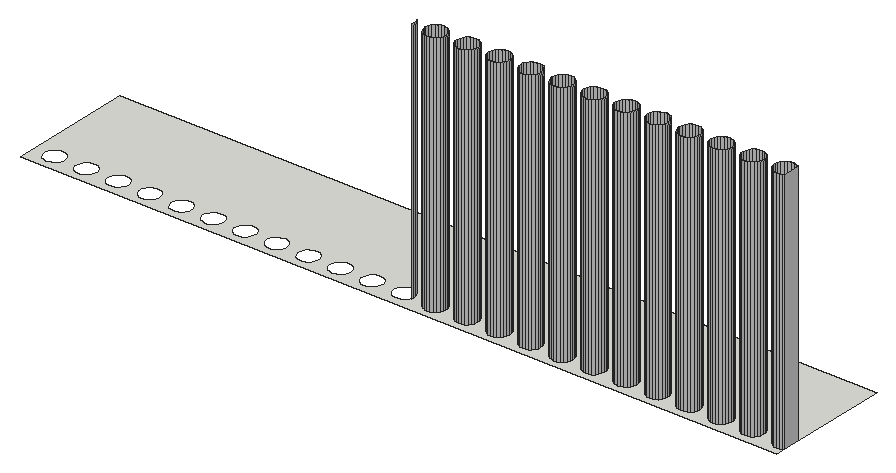
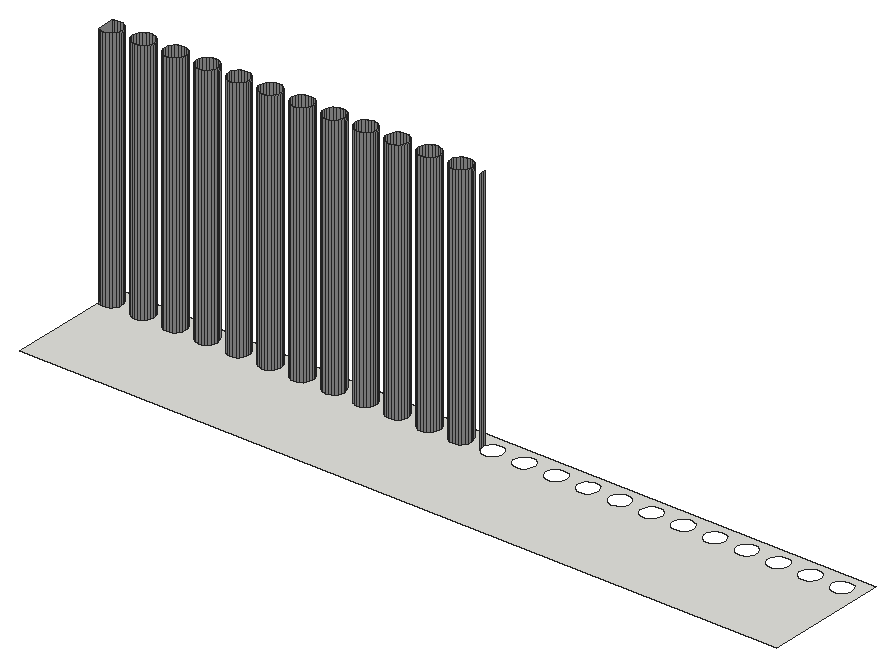
# SketchUp Ruby script. Lengths in millimetres.
U = 1.mm
M = Sketchup.active_model
def pt(a) = Geom::Point3d.new(a.map { |v| v * U })
def face(e, loops, mat)
  f = e.add_face(loops[0].map { |a| pt(a) })
  loops[1..].each { |l| e.add_face(l.map { |a| pt(a) }).erase! }
  f.material = f.back_material = mat if mat
  f
end
# faces: each face lists its corners as indices into pts; further lists are holes
def faces(e, pts, list, mat = nil) = list.each { |f| face(e, (f[0].is_a?(Array) ? f : [f]).map { |l| l.map { |i| pts[i] } }, mat) }
# xy, xz, yz: faces in a plane at the given z, y or x. An outline is a flat list of corners, or four numbers for a rectangle; further outlines are holes
def ring(l) = l.size == 4 ? [[l[0], l[1]], [l[2], l[1]], [l[2], l[3]], [l[0], l[3]]] : l.each_slice(2).to_a
def flat(e, list, mat, &to3) = list.each { |f| face(e, (f[0].is_a?(Array) ? f : [f]).map { |l| ring(l).map { |u, v| to3.(u, v) } }, mat) }
def xy(e, z, list, mat = nil) = flat(e, list, mat) { |x, y| [x, y, z] }
def xz(e, y, list, mat = nil) = flat(e, list, mat) { |x, z| [x, y, z] }
def yz(e, x, list, mat = nil) = flat(e, list, mat) { |y, z| [x, y, z] }
def lines(e, pts, list) = list.each { |a, b| e.add_line(pt(pts[a]), pt(pts[b])) }
# prism: a flat outline (further loops are holes) pulled along v
def prism(e, loops, v, mat = nil)
  f = face(e, loops, mat); d = Geom::Vector3d.new(v.map { |x| x * U })
  f.pushpull(f.normal.samedirection?(d) ? d.length : -d.length)
end
def box(e, o, s, mat = nil) = prism(e, [[o, [o[0] + s[0], o[1], o[2]], [o[0] + s[0], o[1] + s[1], o[2]], [o[0], o[1] + s[1], o[2]]]], [0, 0, s[2]], mat)
def at(x, y, z, deg = 0) = Geom::Transformation.translation(pt([x, y, z])) * Geom::Transformation.rotation(ORIGIN, Z_AXIS, deg.degrees)
def axes(o, x, y, z) = Geom::Transformation.new([*x, 0, *y, 0, *z, 0, *pt(o).to_a, 1])
def part(name) = M.definitions.add(name)
# library, detail: a bought-in or finely detailed component or shape, given as its bounding box
def library(name, o, s) = part(name).tap { |d| box(d.entities, o, s) }
def detail(e, o, s) = box(e.add_group.entities, o, s)
def put(e, d, t, mat = nil) = e.add_instance(d, t).tap { |i| i.material = mat if mat }
def group(e, t, mat = nil) = e.add_group.tap { |g| g.transformation = t; g.material = mat if mat }.entities
root = M.entities
M.materials.add("[Metal Corrugated Shiny]").color = [193, 193, 193]
xy(root,3899.4,[[[7199.4,887.4,11890.5,887.4,11890.5,946.6,11883.2,941.2,11867.4,934.9,11850.5,932.9,11833.7,935.4,11818.1,942.1,11804.8,952.6,11794.6,966.2,11788.3,982,11786.4,998.9,11788.8,1015.7,11795.5,1031.3,11806.1,1044.7,11819.7,1054.8,11835.5,1061.1,11852.3,1063.1,11869.2,1060.6,11884.8,1053.9,11890.5,1049.4,11890.5,1657.4,7199.4,1657.4],[11063.1,932.9,11046.3,935.4,11030.7,942.1,11017.4,952.6,11007.2,966.2,11000.9,982,10999,998.9,11001.4,1015.7,11008.1,1031.3,11018.7,1044.7,11032.3,1054.8,11048.1,1061.1,11064.9,1063.1,11081.8,1060.6,11097.4,1053.9,11110.7,1043.4,11120.9,1029.8,11127.1,1014,11129.1,997.1,11126.7,980.3,11120,964.7,11109.4,951.3,11095.8,941.2,11080,934.9],[11653.7,932.9,11636.9,935.4,11621.3,942.1,11607.9,952.6,11597.8,966.2,11591.5,982,11589.5,998.9,11592,1015.7,11598.7,1031.3,11609.2,1044.7,11622.8,1054.8,11638.6,1061.1,11655.5,1063.1,11672.3,1060.6,11687.9,1053.9,11701.3,1043.4,11711.4,1029.8,11717.7,1014,11719.7,997.1,11717.2,980.3,11710.5,964.7,11700,951.3,11686.4,941.2,11670.6,934.9],[11260,932.9,11243.2,935.4,11227.6,942.1,11214.2,952.6,11204.1,966.2,11197.8,982,11195.8,998.9,11198.3,1015.7,11205,1031.3,11215.5,1044.7,11229.1,1054.8,11244.9,1061.1,11261.8,1063.1,11278.6,1060.6,11294.2,1053.9,11307.6,1043.4,11317.7,1029.8,11324,1014,11326,997.1,11323.5,980.3,11316.8,964.7,11306.3,951.3,11292.7,941.2,11276.9,934.9],[10669.4,932.9,10652.6,935.4,10637,942.1,10623.7,952.6,10613.5,966.2,10607.2,982,10605.3,998.9,10607.7,1015.7,10614.4,1031.3,10625,1044.7,10638.6,1054.8,10654.4,1061.1,10671.2,1063.1,10688.1,1060.6,10703.7,1053.9,10717,1043.4,10727.2,1029.8,10733.4,1014,10735.4,997.1,10733,980.3,10726.3,964.7,10715.7,951.3,10702.1,941.2,10686.3,934.9],[8110.4,932.9,8093.6,935.4,8078,942.1,8064.6,952.6,8054.5,966.2,8048.2,982,8046.2,998.9,8048.7,1015.7,8055.4,1031.3,8065.9,1044.7,8079.5,1054.8,8095.3,1061.1,8112.2,1063.1,8129,1060.6,8144.6,1053.9,8158,1043.4,8168.1,1029.8,8174.4,1014,8176.4,997.1,8173.9,980.3,8167.2,964.7,8156.7,951.3,8143.1,941.2,8127.3,934.9],[9882,932.9,9865.2,935.4,9849.6,942.1,9836.3,952.6,9826.1,966.2,9819.8,982,9817.9,998.9,9820.3,1015.7,9827,1031.3,9837.6,1044.7,9851.2,1054.8,9867,1061.1,9883.8,1063.1,9900.7,1060.6,9916.3,1053.9,9929.6,1043.4,9939.8,1029.8,9946,1014,9948,997.1,9945.6,980.3,9938.9,964.7,9928.3,951.3,9914.7,941.2,9898.9,934.9],[11456.8,932.9,11440,935.4,11424.4,942.1,11411.1,952.6,11400.9,966.2,11394.6,982,11392.7,998.9,11395.1,1015.7,11401.8,1031.3,11412.4,1044.7,11426,1054.8,11441.8,1061.1,11458.6,1063.1,11475.5,1060.6,11491.1,1053.9,11504.4,1043.4,11514.6,1029.8,11520.8,1014,11522.8,997.1,11520.4,980.3,11513.7,964.7,11503.1,951.3,11489.5,941.2,11473.7,934.9],[7323,932.9,7306.2,935.4,7290.6,942.1,7277.2,952.6,7267.1,966.2,7260.8,982,7258.8,998.9,7261.3,1015.7,7268,1031.3,7278.5,1044.7,7292.1,1054.8,7307.9,1061.1,7324.8,1063.1,7341.6,1060.6,7357.2,1053.9,7370.6,1043.4,7380.7,1029.8,7387,1014,7389,997.1,7386.5,980.3,7379.8,964.7,7369.3,951.3,7355.7,941.2,7339.9,934.9],[7716.7,932.9,7699.9,935.4,7684.3,942.1,7670.9,952.6,7660.8,966.2,7654.5,982,7652.5,998.9,7655,1015.7,7661.7,1031.3,7672.2,1044.7,7685.8,1054.8,7701.6,1061.1,7718.5,1063.1,7735.3,1060.6,7750.9,1053.9,7764.3,1043.4,7774.4,1029.8,7780.7,1014,7782.7,997.1,7780.2,980.3,7773.5,964.7,7763,951.3,7749.4,941.2,7733.6,934.9],[7913.5,932.9,7896.7,935.4,7881.1,942.1,7867.8,952.6,7857.6,966.2,7851.3,982,7849.4,998.9,7851.8,1015.7,7858.5,1031.3,7869.1,1044.7,7882.7,1054.8,7898.5,1061.1,7915.3,1063.1,7932.2,1060.6,7947.8,1053.9,7961.1,1043.4,7971.3,1029.8,7977.5,1014,7979.5,997.1,7977.1,980.3,7970.4,964.7,7959.8,951.3,7946.2,941.2,7930.4,934.9],[8897.8,932.9,8881,935.4,8865.4,942.1,8852,952.6,8841.9,966.2,8835.6,982,8833.6,998.9,8836.1,1015.7,8842.8,1031.3,8853.3,1044.7,8866.9,1054.8,8882.7,1061.1,8899.6,1063.1,8916.4,1060.6,8932,1053.9,8945.4,1043.4,8955.5,1029.8,8961.8,1014,8963.8,997.1,8961.3,980.3,8954.6,964.7,8944.1,951.3,8930.5,941.2,8914.7,934.9],[9094.6,932.9,9077.8,935.4,9062.2,942.1,9048.9,952.6,9038.7,966.2,9032.4,982,9030.5,998.9,9032.9,1015.7,9039.6,1031.3,9050.2,1044.7,9063.8,1054.8,9079.6,1061.1,9096.4,1063.1,9113.3,1060.6,9128.9,1053.9,9142.2,1043.4,9152.4,1029.8,9158.6,1014,9160.6,997.1,9158.2,980.3,9151.5,964.7,9140.9,951.3,9127.3,941.2,9111.5,934.9],[7519.8,932.9,7503,935.4,7487.4,942.1,7474.1,952.6,7463.9,966.2,7457.6,982,7455.7,998.9,7458.1,1015.7,7464.8,1031.3,7475.4,1044.7,7489,1054.8,7504.8,1061.1,7521.6,1063.1,7538.5,1060.6,7554.1,1053.9,7567.4,1043.4,7577.6,1029.8,7583.8,1014,7585.8,997.1,7583.4,980.3,7576.7,964.7,7566.1,951.3,7552.5,941.2,7536.7,934.9],[8504.1,932.9,8487.3,935.4,8471.7,942.1,8458.3,952.6,8448.2,966.2,8441.9,982,8439.9,998.9,8442.4,1015.7,8449.1,1031.3,8459.6,1044.7,8473.2,1054.8,8489,1061.1,8505.9,1063.1,8522.7,1060.6,8538.3,1053.9,8551.7,1043.4,8561.8,1029.8,8568.1,1014,8570.1,997.1,8567.6,980.3,8560.9,964.7,8550.4,951.3,8536.8,941.2,8521,934.9],[9488.3,932.9,9471.5,935.4,9455.9,942.1,9442.6,952.6,9432.4,966.2,9426.1,982,9424.2,998.9,9426.6,1015.7,9433.3,1031.3,9443.9,1044.7,9457.5,1054.8,9473.3,1061.1,9490.1,1063.1,9507,1060.6,9522.6,1053.9,9535.9,1043.4,9546.1,1029.8,9552.3,1014,9554.3,997.1,9551.9,980.3,9545.2,964.7,9534.6,951.3,9521,941.2,9505.2,934.9],[10472.6,932.9,10455.8,935.4,10440.2,942.1,10426.8,952.6,10416.7,966.2,10410.4,982,10408.4,998.9,10410.9,1015.7,10417.6,1031.3,10428.1,1044.7,10441.7,1054.8,10457.5,1061.1,10474.4,1063.1,10491.2,1060.6,10506.8,1053.9,10520.2,1043.4,10530.3,1029.8,10536.6,1014,10538.6,997.1,10536.1,980.3,10529.4,964.7,10518.9,951.3,10505.3,941.2,10489.5,934.9],[9685.2,932.9,9668.4,935.4,9652.8,942.1,9639.4,952.6,9629.3,966.2,9623,982,9621,998.9,9623.5,1015.7,9630.2,1031.3,9640.7,1044.7,9654.3,1054.8,9670.1,1061.1,9687,1063.1,9703.8,1060.6,9719.4,1053.9,9732.8,1043.4,9742.9,1029.8,9749.2,1014,9751.2,997.1,9748.7,980.3,9742,964.7,9731.5,951.3,9717.9,941.2,9702.1,934.9],[8700.9,932.9,8684.1,935.4,8668.5,942.1,8655.2,952.6,8645,966.2,8638.7,982,8636.8,998.9,8639.2,1015.7,8645.9,1031.3,8656.5,1044.7,8670.1,1054.8,8685.9,1061.1,8702.7,1063.1,8719.6,1060.6,8735.2,1053.9,8748.5,1043.4,8758.7,1029.8,8764.9,1014,8766.9,997.1,8764.5,980.3,8757.8,964.7,8747.2,951.3,8733.6,941.2,8717.8,934.9],[10078.9,932.9,10062.1,935.4,10046.5,942.1,10033.1,952.6,10023,966.2,10016.7,982,10014.7,998.9,10017.2,1015.7,10023.9,1031.3,10034.4,1044.7,10048,1054.8,10063.8,1061.1,10080.7,1063.1,10097.5,1060.6,10113.1,1053.9,10126.5,1043.4,10136.6,1029.8,10142.9,1014,10144.9,997.1,10142.4,980.3,10135.7,964.7,10125.2,951.3,10111.6,941.2,10095.8,934.9],[8307.2,932.9,8290.4,935.4,8274.8,942.1,8261.5,952.6,8251.3,966.2,8245,982,8243.1,998.9,8245.5,1015.7,8252.2,1031.3,8262.8,1044.7,8276.4,1054.8,8292.2,1061.1,8309,1063.1,8325.9,1060.6,8341.5,1053.9,8354.8,1043.4,8365,1029.8,8371.2,1014,8373.2,997.1,8370.8,980.3,8364.1,964.7,8353.5,951.3,8339.9,941.2,8324.1,934.9],[9291.5,932.9,9274.7,935.4,9259.1,942.1,9245.7,952.6,9235.6,966.2,9229.3,982,9227.3,998.9,9229.8,1015.7,9236.5,1031.3,9247,1044.7,9260.6,1054.8,9276.4,1061.1,9293.3,1063.1,9310.1,1060.6,9325.7,1053.9,9339.1,1043.4,9349.2,1029.8,9355.5,1014,9357.5,997.1,9355,980.3,9348.3,964.7,9337.8,951.3,9324.2,941.2,9308.4,934.9],[10275.7,932.9,10258.9,935.4,10243.3,942.1,10230,952.6,10219.8,966.2,10213.5,982,10211.6,998.9,10214,1015.7,10220.7,1031.3,10231.3,1044.7,10244.9,1054.8,10260.7,1061.1,10277.5,1063.1,10294.4,1060.6,10310,1053.9,10323.3,1043.4,10333.5,1029.8,10339.7,1014,10341.7,997.1,10339.3,980.3,10332.6,964.7,10322,951.3,10308.4,941.2,10292.6,934.9],[10866.3,932.9,10849.5,935.4,10833.9,942.1,10820.5,952.6,10810.4,966.2,10804.1,982,10802.1,998.9,10804.6,1015.7,10811.3,1031.3,10821.8,1044.7,10835.4,1054.8,10851.2,1061.1,10868.1,1063.1,10884.9,1060.6,10900.5,1053.9,10913.9,1043.4,10924,1029.8,10930.3,1014,10932.3,997.1,10929.8,980.3,10923.1,964.7,10912.6,951.3,10899,941.2,10883.2,934.9]]])
xy(root,3899.4,[[9685.2,932.9,9668.4,935.4,9652.8,942.1,9639.4,952.6,9629.3,966.2,9623,982,9621,998.9,9623.5,1015.7,9630.2,1031.3,9640.7,1044.7,9654.3,1054.8,9670.1,1061.1,9687,1063.1,9703.8,1060.6,9719.4,1053.9,9732.8,1043.4,9742.9,1029.8,9749.2,1014,9751.2,997.1,9748.7,980.3,9742,964.7,9731.5,951.3,9717.9,941.2,9702.1,934.9],[9882,932.9,9865.2,935.4,9849.6,942.1,9836.3,952.6,9826.1,966.2,9819.8,982,9817.9,998.9,9820.3,1015.7,9827,1031.3,9837.6,1044.7,9851.2,1054.8,9867,1061.1,9883.8,1063.1,9900.7,1060.6,9916.3,1053.9,9929.6,1043.4,9939.8,1029.8,9946,1014,9948,997.1,9945.6,980.3,9938.9,964.7,9928.3,951.3,9914.7,941.2,9898.9,934.9],[10078.9,932.9,10062.1,935.4,10046.5,942.1,10033.1,952.6,10023,966.2,10016.7,982,10014.7,998.9,10017.2,1015.7,10023.9,1031.3,10034.4,1044.7,10048,1054.8,10063.8,1061.1,10080.7,1063.1,10097.5,1060.6,10113.1,1053.9,10126.5,1043.4,10136.6,1029.8,10142.9,1014,10144.9,997.1,10142.4,980.3,10135.7,964.7,10125.2,951.3,10111.6,941.2,10095.8,934.9],[10275.7,932.9,10258.9,935.4,10243.3,942.1,10230,952.6,10219.8,966.2,10213.5,982,10211.6,998.9,10214,1015.7,10220.7,1031.3,10231.3,1044.7,10244.9,1054.8,10260.7,1061.1,10277.5,1063.1,10294.4,1060.6,10310,1053.9,10323.3,1043.4,10333.5,1029.8,10339.7,1014,10341.7,997.1,10339.3,980.3,10332.6,964.7,10322,951.3,10308.4,941.2,10292.6,934.9],[10472.6,932.9,10455.8,935.4,10440.2,942.1,10426.8,952.6,10416.7,966.2,10410.4,982,10408.4,998.9,10410.9,1015.7,10417.6,1031.3,10428.1,1044.7,10441.7,1054.8,10457.5,1061.1,10474.4,1063.1,10491.2,1060.6,10506.8,1053.9,10520.2,1043.4,10530.3,1029.8,10536.6,1014,10538.6,997.1,10536.1,980.3,10529.4,964.7,10518.9,951.3,10505.3,941.2,10489.5,934.9],
  [10669.4,932.9,10652.6,935.4,10637,942.1,10623.7,952.6,10613.5,966.2,10607.2,982,10605.3,998.9,10607.7,1015.7,10614.4,1031.3,10625,1044.7,10638.6,1054.8,10654.4,1061.1,10671.2,1063.1,10688.1,1060.6,10703.7,1053.9,10717,1043.4,10727.2,1029.8,10733.4,1014,10735.4,997.1,10733,980.3,10726.3,964.7,10715.7,951.3,10702.1,941.2,10686.3,934.9],[10866.3,932.9,10849.5,935.4,10833.9,942.1,10820.5,952.6,10810.4,966.2,10804.1,982,10802.1,998.9,10804.6,1015.7,10811.3,1031.3,10821.8,1044.7,10835.4,1054.8,10851.2,1061.1,10868.1,1063.1,10884.9,1060.6,10900.5,1053.9,10913.9,1043.4,10924,1029.8,10930.3,1014,10932.3,997.1,10929.8,980.3,10923.1,964.7,10912.6,951.3,10899,941.2,10883.2,934.9],[11063.1,932.9,11046.3,935.4,11030.7,942.1,11017.4,952.6,11007.2,966.2,11000.9,982,10999,998.9,11001.4,1015.7,11008.1,1031.3,11018.7,1044.7,11032.3,1054.8,11048.1,1061.1,11064.9,1063.1,11081.8,1060.6,11097.4,1053.9,11110.7,1043.4,11120.9,1029.8,11127.1,1014,11129.1,997.1,11126.7,980.3,11120,964.7,11109.4,951.3,11095.8,941.2,11080,934.9],[11260,932.9,11243.2,935.4,11227.6,942.1,11214.2,952.6,11204.1,966.2,11197.8,982,11195.8,998.9,11198.3,1015.7,11205,1031.3,11215.5,1044.7,11229.1,1054.8,11244.9,1061.1,11261.8,1063.1,11278.6,1060.6,11294.2,1053.9,11307.6,1043.4,11317.7,1029.8,11324,1014,11326,997.1,11323.5,980.3,11316.8,964.7,11306.3,951.3,11292.7,941.2,11276.9,934.9],[11456.8,932.9,11440,935.4,11424.4,942.1,11411.1,952.6,11400.9,966.2,11394.6,982,11392.7,998.9,11395.1,1015.7,11401.8,1031.3,11412.4,1044.7,11426,1054.8,11441.8,1061.1,11458.6,1063.1,11475.5,1060.6,11491.1,1053.9,11504.4,1043.4,11514.6,1029.8,11520.8,1014,11522.8,997.1,11520.4,980.3,11513.7,964.7,11503.1,951.3,11489.5,941.2,11473.7,934.9],
  [11653.7,932.9,11636.9,935.4,11621.3,942.1,11607.9,952.6,11597.8,966.2,11591.5,982,11589.5,998.9,11592,1015.7,11598.7,1031.3,11609.2,1044.7,11622.8,1054.8,11638.6,1061.1,11655.5,1063.1,11672.3,1060.6,11687.9,1053.9,11701.3,1043.4,11711.4,1029.8,11717.7,1014,11719.7,997.1,11717.2,980.3,11710.5,964.7,11700,951.3,11686.4,941.2,11670.6,934.9],[11850.5,932.9,11833.7,935.4,11818.1,942.1,11804.8,952.6,11794.6,966.2,11788.3,982,11786.4,998.9,11788.8,1015.7,11795.5,1031.3,11806.1,1044.7,11819.7,1054.8,11835.5,1061.1,11852.3,1063.1,11869.2,1060.6,11884.8,1053.9,11890.5,1049.4,11890.5,946.6,11883.2,941.2,11867.4,934.9]],"[Metal Corrugated Shiny]")
yz(root,11890.5,[[946.6,3899.4,1049.4,5423.4]],"[Metal Corrugated Shiny]")
p = [[9668.4,935.4,3899.4],[9685.2,932.9,3899.4],[9685.2,932.9,5423.4],[9668.4,935.4,5423.4],[9702.1,934.9,3899.4],[9702.1,934.9,5423.4],
  [9865.2,935.4,3899.4],[9882,932.9,3899.4],[9882,932.9,5423.4],[9865.2,935.4,5423.4],[9898.9,934.9,3899.4],[9898.9,934.9,5423.4],
  [10062.1,935.4,3899.4],[10078.9,932.9,3899.4],[10078.9,932.9,5423.4],[10062.1,935.4,5423.4],[10095.8,934.9,3899.4],[10095.8,934.9,5423.4],
  [10258.9,935.4,3899.4],[10275.7,932.9,3899.4],[10275.7,932.9,5423.4],[10258.9,935.4,5423.4],[10292.6,934.9,3899.4],[10292.6,934.9,5423.4],
  [10455.8,935.4,3899.4],[10472.6,932.9,3899.4],[10472.6,932.9,5423.4],[10455.8,935.4,5423.4],[10489.5,934.9,3899.4],[10489.5,934.9,5423.4],
  [10652.6,935.4,3899.4],[10669.4,932.9,3899.4],[10669.4,932.9,5423.4],[10652.6,935.4,5423.4],[10686.3,934.9,3899.4],[10686.3,934.9,5423.4],
  [10849.5,935.4,3899.4],[10866.3,932.9,3899.4],[10866.3,932.9,5423.4],[10849.5,935.4,5423.4],[10883.2,934.9,3899.4],[10883.2,934.9,5423.4],
  [11046.3,935.4,3899.4],[11063.1,932.9,3899.4],[11063.1,932.9,5423.4],[11046.3,935.4,5423.4],[11080,934.9,3899.4],[11080,934.9,5423.4],
  [11243.2,935.4,3899.4],[11260,932.9,3899.4],[11260,932.9,5423.4],[11243.2,935.4,5423.4],[11276.9,934.9,3899.4],[11276.9,934.9,5423.4],
  [11440,935.4,3899.4],[11456.8,932.9,3899.4],[11456.8,932.9,5423.4],[11440,935.4,5423.4],[11473.7,934.9,3899.4],[11473.7,934.9,5423.4],
  [11636.9,935.4,3899.4],[11653.7,932.9,3899.4],[11653.7,932.9,5423.4],[11636.9,935.4,5423.4],[11670.6,934.9,3899.4],[11670.6,934.9,5423.4],
  [11833.7,935.4,3899.4],[11850.5,932.9,3899.4],[11850.5,932.9,5423.4],[11833.7,935.4,5423.4],[11867.4,934.9,3899.4],[11867.4,934.9,5423.4],
  [9717.9,941.2,3899.4],[9717.9,941.2,5423.4],[9914.7,941.2,3899.4],[9914.7,941.2,5423.4],[10111.6,941.2,3899.4],[10111.6,941.2,5423.4],
  [10308.4,941.2,3899.4],[10308.4,941.2,5423.4],[10505.3,941.2,3899.4],[10505.3,941.2,5423.4],[10702.1,941.2,3899.4],[10702.1,941.2,5423.4],
  [10899,941.2,3899.4],[10899,941.2,5423.4],[11095.8,941.2,3899.4],[11095.8,941.2,5423.4],[11292.7,941.2,3899.4],[11292.7,941.2,5423.4],
  [11489.5,941.2,3899.4],[11489.5,941.2,5423.4],[11686.4,941.2,3899.4],[11686.4,941.2,5423.4],[11883.2,941.2,3899.4],[11883.2,941.2,5423.4],
  [9652.8,942.1,3899.4],[9652.8,942.1,5423.4],[9849.6,942.1,3899.4],[9849.6,942.1,5423.4],[10046.5,942.1,3899.4],[10046.5,942.1,5423.4],
  [10243.3,942.1,3899.4],[10243.3,942.1,5423.4],[10440.2,942.1,3899.4],[10440.2,942.1,5423.4],[10637,942.1,3899.4],[10637,942.1,5423.4],
  [10833.9,942.1,3899.4],[10833.9,942.1,5423.4],[11030.7,942.1,3899.4],[11030.7,942.1,5423.4],[11227.6,942.1,3899.4],[11227.6,942.1,5423.4],
  [11424.4,942.1,3899.4],[11424.4,942.1,5423.4],[11621.3,942.1,3899.4],[11621.3,942.1,5423.4],[11818.1,942.1,3899.4],[11818.1,942.1,5423.4],
  [9731.5,951.3,3899.4],[9731.5,951.3,5423.4],[9928.3,951.3,3899.4],[9928.3,951.3,5423.4],[10125.2,951.3,3899.4],[10125.2,951.3,5423.4],
  [10322,951.3,3899.4],[10322,951.3,5423.4],[10518.9,951.3,3899.4],[10518.9,951.3,5423.4],[10715.7,951.3,3899.4],[10715.7,951.3,5423.4],
  [10912.6,951.3,3899.4],[10912.6,951.3,5423.4],[11109.4,951.3,3899.4],[11109.4,951.3,5423.4],[11306.3,951.3,3899.4],[11306.3,951.3,5423.4],
  [11503.1,951.3,3899.4],[11503.1,951.3,5423.4],[11700,951.3,3899.4],[11700,951.3,5423.4],[11890.5,946.6,3899.4],[11890.5,946.6,5423.4],
  [9639.4,952.6,3899.4],[9639.4,952.6,5423.4],[9836.3,952.6,3899.4],[9836.3,952.6,5423.4],[10033.1,952.6,3899.4],[10033.1,952.6,5423.4],
  [10230,952.6,3899.4],[10230,952.6,5423.4],[10426.8,952.6,3899.4],[10426.8,952.6,5423.4],[10623.7,952.6,3899.4],[10623.7,952.6,5423.4],
  [10820.5,952.6,3899.4],[10820.5,952.6,5423.4],[11017.4,952.6,3899.4],[11017.4,952.6,5423.4],[11214.2,952.6,3899.4],[11214.2,952.6,5423.4],
  [11411.1,952.6,3899.4],[11411.1,952.6,5423.4],[11607.9,952.6,3899.4],[11607.9,952.6,5423.4],[11804.8,952.6,3899.4],[11804.8,952.6,5423.4],
  [9742,964.7,3899.4],[9742,964.7,5423.4],[9938.9,964.7,3899.4],[9938.9,964.7,5423.4],[10135.7,964.7,3899.4],[10135.7,964.7,5423.4],
  [10332.6,964.7,3899.4],[10332.6,964.7,5423.4],[10529.4,964.7,3899.4],[10529.4,964.7,5423.4],[10726.3,964.7,3899.4],[10726.3,964.7,5423.4],
  [10923.1,964.7,3899.4],[10923.1,964.7,5423.4],[11120,964.7,3899.4],[11120,964.7,5423.4],[11316.8,964.7,3899.4],[11316.8,964.7,5423.4],
  [11513.7,964.7,3899.4],[11513.7,964.7,5423.4],[11710.5,964.7,3899.4],[11710.5,964.7,5423.4],[9629.3,966.2,3899.4],[9629.3,966.2,5423.4],
  [9826.1,966.2,3899.4],[9826.1,966.2,5423.4],[10023,966.2,3899.4],[10023,966.2,5423.4],[10219.8,966.2,3899.4],[10219.8,966.2,5423.4],
  [10416.7,966.2,3899.4],[10416.7,966.2,5423.4],[10613.5,966.2,3899.4],[10613.5,966.2,5423.4],[10810.4,966.2,3899.4],[10810.4,966.2,5423.4],
  [11007.2,966.2,3899.4],[11007.2,966.2,5423.4],[11204.1,966.2,3899.4],[11204.1,966.2,5423.4],[11400.9,966.2,3899.4],[11400.9,966.2,5423.4],
  [11597.8,966.2,3899.4],[11597.8,966.2,5423.4],[11794.6,966.2,3899.4],[11794.6,966.2,5423.4],[9748.7,980.3,3899.4],[9748.7,980.3,5423.4],
  [9945.6,980.3,3899.4],[9945.6,980.3,5423.4],[10142.4,980.3,3899.4],[10142.4,980.3,5423.4],[10339.3,980.3,3899.4],[10339.3,980.3,5423.4],
  [10536.1,980.3,3899.4],[10536.1,980.3,5423.4],[10733,980.3,3899.4],[10733,980.3,5423.4],[10929.8,980.3,3899.4],[10929.8,980.3,5423.4],
  [11126.7,980.3,3899.4],[11126.7,980.3,5423.4],[11323.5,980.3,3899.4],[11323.5,980.3,5423.4],[11520.4,980.3,3899.4],[11520.4,980.3,5423.4],
  [11717.2,980.3,3899.4],[11717.2,980.3,5423.4],[9623,982,3899.4],[9623,982,5423.4],[9819.8,982,3899.4],[9819.8,982,5423.4],
  [10016.7,982,3899.4],[10016.7,982,5423.4],[10213.5,982,3899.4],[10213.5,982,5423.4],[10410.4,982,3899.4],[10410.4,982,5423.4],
  [10607.2,982,3899.4],[10607.2,982,5423.4],[10804.1,982,3899.4],[10804.1,982,5423.4],[11000.9,982,3899.4],[11000.9,982,5423.4],
  [11197.8,982,3899.4],[11197.8,982,5423.4],[11394.6,982,3899.4],[11394.6,982,5423.4],[11591.5,982,3899.4],[11591.5,982,5423.4],
  [11788.3,982,3899.4],[11788.3,982,5423.4],[9551.9,980.3,3899.4],[9554.3,997.1,3899.4],[9554.3,997.1,5423.4],[9551.9,980.3,5423.4],
  [9751.2,997.1,3899.4],[9751.2,997.1,5423.4],[9948,997.1,3899.4],[9948,997.1,5423.4],[10144.9,997.1,3899.4],[10144.9,997.1,5423.4],
  [10341.7,997.1,3899.4],[10341.7,997.1,5423.4],[10538.6,997.1,3899.4],[10538.6,997.1,5423.4],[10735.4,997.1,3899.4],[10735.4,997.1,5423.4],
  [10932.3,997.1,3899.4],[10932.3,997.1,5423.4],[11129.1,997.1,3899.4],[11129.1,997.1,5423.4],[11326,997.1,3899.4],[11326,997.1,5423.4],
  [11522.8,997.1,3899.4],[11522.8,997.1,5423.4],[11719.7,997.1,3899.4],[11719.7,997.1,5423.4],[9621,998.9,3899.4],[9621,998.9,5423.4],
  [9817.9,998.9,3899.4],[9817.9,998.9,5423.4],[10014.7,998.9,3899.4],[10014.7,998.9,5423.4],[10211.6,998.9,3899.4],[10211.6,998.9,5423.4],
  [10408.4,998.9,3899.4],[10408.4,998.9,5423.4],[10605.3,998.9,3899.4],[10605.3,998.9,5423.4],[10802.1,998.9,3899.4],[10802.1,998.9,5423.4],
  [10999,998.9,3899.4],[10999,998.9,5423.4],[11195.8,998.9,3899.4],[11195.8,998.9,5423.4],[11392.7,998.9,3899.4],[11392.7,998.9,5423.4],
  [11589.5,998.9,3899.4],[11589.5,998.9,5423.4],[11786.4,998.9,3899.4],[11786.4,998.9,5423.4],[9552.3,1014,3899.4],[9552.3,1014,5423.4],
  [9749.2,1014,3899.4],[9749.2,1014,5423.4],[9946,1014,3899.4],[9946,1014,5423.4],[10142.9,1014,3899.4],[10142.9,1014,5423.4],
  [10339.7,1014,3899.4],[10339.7,1014,5423.4],[10536.6,1014,3899.4],[10536.6,1014,5423.4],[10733.4,1014,3899.4],[10733.4,1014,5423.4],
  [10930.3,1014,3899.4],[10930.3,1014,5423.4],[11127.1,1014,3899.4],[11127.1,1014,5423.4],[11324,1014,3899.4],[11324,1014,5423.4],
  [11520.8,1014,3899.4],[11520.8,1014,5423.4],[11717.7,1014,3899.4],[11717.7,1014,5423.4],[9623.5,1015.7,3899.4],[9623.5,1015.7,5423.4],
  [9820.3,1015.7,3899.4],[9820.3,1015.7,5423.4],[10017.2,1015.7,3899.4],[10017.2,1015.7,5423.4],[10214,1015.7,3899.4],[10214,1015.7,5423.4],
  [10410.9,1015.7,3899.4],[10410.9,1015.7,5423.4],[10607.7,1015.7,3899.4],[10607.7,1015.7,5423.4],[10804.6,1015.7,3899.4],[10804.6,1015.7,5423.4],
  [11001.4,1015.7,3899.4],[11001.4,1015.7,5423.4],[11198.3,1015.7,3899.4],[11198.3,1015.7,5423.4],[11395.1,1015.7,3899.4],[11395.1,1015.7,5423.4],
  [11592,1015.7,3899.4],[11592,1015.7,5423.4],[11788.8,1015.7,3899.4],[11788.8,1015.7,5423.4],[9546.1,1029.8,3899.4],[9546.1,1029.8,5423.4],
  [9742.9,1029.8,3899.4],[9742.9,1029.8,5423.4],[9939.8,1029.8,3899.4],[9939.8,1029.8,5423.4],[10136.6,1029.8,3899.4],[10136.6,1029.8,5423.4],
  [10333.5,1029.8,3899.4],[10333.5,1029.8,5423.4],[10530.3,1029.8,3899.4],[10530.3,1029.8,5423.4],[10727.2,1029.8,3899.4],[10727.2,1029.8,5423.4],
  [10924,1029.8,3899.4],[10924,1029.8,5423.4],[11120.9,1029.8,3899.4],[11120.9,1029.8,5423.4],[11317.7,1029.8,3899.4],[11317.7,1029.8,5423.4],
  [11514.6,1029.8,3899.4],[11514.6,1029.8,5423.4],[11711.4,1029.8,3899.4],[11711.4,1029.8,5423.4],[9630.2,1031.3,3899.4],[9630.2,1031.3,5423.4],
  [9827,1031.3,3899.4],[9827,1031.3,5423.4],[10023.9,1031.3,3899.4],[10023.9,1031.3,5423.4],[10220.7,1031.3,3899.4],[10220.7,1031.3,5423.4],
  [10417.6,1031.3,3899.4],[10417.6,1031.3,5423.4],[10614.4,1031.3,3899.4],[10614.4,1031.3,5423.4],[10811.3,1031.3,3899.4],[10811.3,1031.3,5423.4],
  [11008.1,1031.3,3899.4],[11008.1,1031.3,5423.4],[11205,1031.3,3899.4],[11205,1031.3,5423.4],[11401.8,1031.3,3899.4],[11401.8,1031.3,5423.4],
  [11598.7,1031.3,3899.4],[11598.7,1031.3,5423.4],[11795.5,1031.3,3899.4],[11795.5,1031.3,5423.4],[9732.8,1043.4,3899.4],[9732.8,1043.4,5423.4],
  [9929.6,1043.4,3899.4],[9929.6,1043.4,5423.4],[10126.5,1043.4,3899.4],[10126.5,1043.4,5423.4],[10323.3,1043.4,3899.4],[10323.3,1043.4,5423.4],
  [10520.2,1043.4,3899.4],[10520.2,1043.4,5423.4],[10717,1043.4,3899.4],[10717,1043.4,5423.4],[10913.9,1043.4,3899.4],[10913.9,1043.4,5423.4],
  [11110.7,1043.4,3899.4],[11110.7,1043.4,5423.4],[11307.6,1043.4,3899.4],[11307.6,1043.4,5423.4],[11504.4,1043.4,3899.4],[11504.4,1043.4,5423.4],
  [11701.3,1043.4,3899.4],[11701.3,1043.4,5423.4],[9640.7,1044.7,3899.4],[9640.7,1044.7,5423.4],[9837.6,1044.7,3899.4],[9837.6,1044.7,5423.4],
  [10034.4,1044.7,3899.4],[10034.4,1044.7,5423.4],[10231.3,1044.7,3899.4],[10231.3,1044.7,5423.4],[10428.1,1044.7,3899.4],[10428.1,1044.7,5423.4],
  [10625,1044.7,3899.4],[10625,1044.7,5423.4],[10821.8,1044.7,3899.4],[10821.8,1044.7,5423.4],[11018.7,1044.7,3899.4],[11018.7,1044.7,5423.4],
  [11215.5,1044.7,3899.4],[11215.5,1044.7,5423.4],[11412.4,1044.7,3899.4],[11412.4,1044.7,5423.4],[11609.2,1044.7,3899.4],[11609.2,1044.7,5423.4],
  [11806.1,1044.7,3899.4],[11806.1,1044.7,5423.4],[9719.4,1053.9,3899.4],[9719.4,1053.9,5423.4],[9916.3,1053.9,3899.4],[9916.3,1053.9,5423.4],
  [10113.1,1053.9,3899.4],[10113.1,1053.9,5423.4],[10310,1053.9,3899.4],[10310,1053.9,5423.4],[10506.8,1053.9,3899.4],[10506.8,1053.9,5423.4],
  [10703.7,1053.9,3899.4],[10703.7,1053.9,5423.4],[10900.5,1053.9,3899.4],[10900.5,1053.9,5423.4],[11097.4,1053.9,3899.4],[11097.4,1053.9,5423.4],
  [11294.2,1053.9,3899.4],[11294.2,1053.9,5423.4],[11491.1,1053.9,3899.4],[11491.1,1053.9,5423.4],[11687.9,1053.9,3899.4],[11687.9,1053.9,5423.4],
  [9654.3,1054.8,3899.4],[9654.3,1054.8,5423.4],[9851.2,1054.8,3899.4],[9851.2,1054.8,5423.4],[10048,1054.8,3899.4],[10048,1054.8,5423.4],
  [10244.9,1054.8,3899.4],[10244.9,1054.8,5423.4],[10441.7,1054.8,3899.4],[10441.7,1054.8,5423.4],[10638.6,1054.8,3899.4],[10638.6,1054.8,5423.4],
  [10835.4,1054.8,3899.4],[10835.4,1054.8,5423.4],[11032.3,1054.8,3899.4],[11032.3,1054.8,5423.4],[11229.1,1054.8,3899.4],[11229.1,1054.8,5423.4],
  [11426,1054.8,3899.4],[11426,1054.8,5423.4],[11622.8,1054.8,3899.4],[11622.8,1054.8,5423.4],[11819.7,1054.8,3899.4],[11819.7,1054.8,5423.4],
  [11890.5,1049.4,3899.4],[11884.8,1053.9,3899.4],[11884.8,1053.9,5423.4],[11890.5,1049.4,5423.4],[9703.8,1060.6,3899.4],[9703.8,1060.6,5423.4],
  [9900.7,1060.6,3899.4],[9900.7,1060.6,5423.4],[10097.5,1060.6,3899.4],[10097.5,1060.6,5423.4],[10294.4,1060.6,3899.4],[10294.4,1060.6,5423.4],
  [10491.2,1060.6,3899.4],[10491.2,1060.6,5423.4],[10688.1,1060.6,3899.4],[10688.1,1060.6,5423.4],[10884.9,1060.6,3899.4],[10884.9,1060.6,5423.4],
  [11081.8,1060.6,3899.4],[11081.8,1060.6,5423.4],[11278.6,1060.6,3899.4],[11278.6,1060.6,5423.4],[11475.5,1060.6,3899.4],[11475.5,1060.6,5423.4],
  [11672.3,1060.6,3899.4],[11672.3,1060.6,5423.4],[11869.2,1060.6,3899.4],[11869.2,1060.6,5423.4],[9670.1,1061.1,3899.4],[9670.1,1061.1,5423.4],
  [9867,1061.1,3899.4],[9867,1061.1,5423.4],[10063.8,1061.1,3899.4],[10063.8,1061.1,5423.4],[10260.7,1061.1,3899.4],[10260.7,1061.1,5423.4],
  [10457.5,1061.1,3899.4],[10457.5,1061.1,5423.4],[10654.4,1061.1,3899.4],[10654.4,1061.1,5423.4],[10851.2,1061.1,3899.4],[10851.2,1061.1,5423.4],
  [11048.1,1061.1,3899.4],[11048.1,1061.1,5423.4],[11244.9,1061.1,3899.4],[11244.9,1061.1,5423.4],[11441.8,1061.1,3899.4],[11441.8,1061.1,5423.4],
  [11638.6,1061.1,3899.4],[11638.6,1061.1,5423.4],[11835.5,1061.1,3899.4],[11835.5,1061.1,5423.4],[9687,1063.1,3899.4],[9687,1063.1,5423.4],
  [9883.8,1063.1,3899.4],[9883.8,1063.1,5423.4],[10080.7,1063.1,3899.4],[10080.7,1063.1,5423.4],[10277.5,1063.1,3899.4],[10277.5,1063.1,5423.4],
  [10474.4,1063.1,3899.4],[10474.4,1063.1,5423.4],[10671.2,1063.1,3899.4],[10671.2,1063.1,5423.4],[10868.1,1063.1,3899.4],[10868.1,1063.1,5423.4],
  [11064.9,1063.1,3899.4],[11064.9,1063.1,5423.4],[11261.8,1063.1,3899.4],[11261.8,1063.1,5423.4],[11458.6,1063.1,3899.4],[11458.6,1063.1,5423.4],
  [11655.5,1063.1,3899.4],[11655.5,1063.1,5423.4],[11852.3,1063.1,3899.4],[11852.3,1063.1,5423.4]]
faces(root,p,[[0,1,2,3],[1,4,5,2],[6,7,8,9],[7,10,11,8],[12,13,14,15],[13,16,17,14],[18,19,20,21],[19,22,23,20],
  [24,25,26,27],[25,28,29,26],[30,31,32,33],[31,34,35,32],[36,37,38,39],[37,40,41,38],[42,43,44,45],[43,46,47,44],
  [48,49,50,51],[49,52,53,50],[54,55,56,57],[55,58,59,56],[60,61,62,63],[61,64,65,62],[66,67,68,69],[67,70,71,68],
  [4,72,73,5],[10,74,75,11],[16,76,77,17],[22,78,79,23],[28,80,81,29],[34,82,83,35],[40,84,85,41],[46,86,87,47],
  [52,88,89,53],[58,90,91,59],[64,92,93,65],[70,94,95,71],[96,0,3,97],[98,6,9,99],[100,12,15,101],[102,18,21,103],
  [104,24,27,105],[106,30,33,107],[108,36,39,109],[110,42,45,111],[112,48,51,113],[114,54,57,115],[116,60,63,117],[118,66,69,119],
  [72,120,121,73],[74,122,123,75],[76,124,125,77],[78,126,127,79],[80,128,129,81],[82,130,131,83],[84,132,133,85],[86,134,135,87],
  [88,136,137,89],[90,138,139,91],[92,140,141,93],[94,142,143,95],[144,96,97,145],[146,98,99,147],[148,100,101,149],[150,102,103,151],
  [152,104,105,153],[154,106,107,155],[156,108,109,157],[158,110,111,159],[160,112,113,161],[162,114,115,163],[164,116,117,165],[166,118,119,167],
  [120,168,169,121],[122,170,171,123],[124,172,173,125],[126,174,175,127],[128,176,177,129],[130,178,179,131],[132,180,181,133],[134,182,183,135],
  [136,184,185,137],[138,186,187,139],[140,188,189,141],[190,144,145,191],[192,146,147,193],[194,148,149,195],[196,150,151,197],[198,152,153,199],
  [200,154,155,201],[202,156,157,203],[204,158,159,205],[206,160,161,207],[208,162,163,209],[210,164,165,211],[212,166,167,213],[168,214,215,169],
  [170,216,217,171],[172,218,219,173],[174,220,221,175],[176,222,223,177],[178,224,225,179],[180,226,227,181],[182,228,229,183],[184,230,231,185],
  [186,232,233,187],[188,234,235,189],[236,190,191,237],[238,192,193,239],[240,194,195,241],[242,196,197,243],[244,198,199,245],[246,200,201,247],
  [248,202,203,249],[250,204,205,251],[252,206,207,253],[254,208,209,255],[256,210,211,257],[258,212,213,259],[260,261,262,263],[214,264,265,215],
  [216,266,267,217],[218,268,269,219],[220,270,271,221],[222,272,273,223],[224,274,275,225],[226,276,277,227],[228,278,279,229],[230,280,281,231],
  [232,282,283,233],[234,284,285,235],[286,236,237,287],[288,238,239,289],[290,240,241,291],[292,242,243,293],[294,244,245,295],[296,246,247,297],
  [298,248,249,299],[300,250,251,301],[302,252,253,303],[304,254,255,305],[306,256,257,307],[308,258,259,309],[261,310,311,262],[264,312,313,265],
  [266,314,315,267],[268,316,317,269],[270,318,319,271],[272,320,321,273],[274,322,323,275],[276,324,325,277],[278,326,327,279],[280,328,329,281],
  [282,330,331,283],[284,332,333,285],[334,286,287,335],[336,288,289,337],[338,290,291,339],[340,292,293,341],[342,294,295,343],[344,296,297,345],
  [346,298,299,347],[348,300,301,349],[350,302,303,351],[352,304,305,353],[354,306,307,355],[356,308,309,357],[310,358,359,311],[312,360,361,313],
  [314,362,363,315],[316,364,365,317],[318,366,367,319],[320,368,369,321],[322,370,371,323],[324,372,373,325],[326,374,375,327],[328,376,377,329],
  [330,378,379,331],[332,380,381,333],[382,334,335,383],[384,336,337,385],[386,338,339,387],[388,340,341,389],[390,342,343,391],[392,344,345,393],
  [394,346,347,395],[396,348,349,397],[398,350,351,399],[400,352,353,401],[402,354,355,403],[404,356,357,405],[360,406,407,361],[362,408,409,363],
  [364,410,411,365],[366,412,413,367],[368,414,415,369],[370,416,417,371],[372,418,419,373],[374,420,421,375],[376,422,423,377],[378,424,425,379],
  [380,426,427,381],[428,382,383,429],[430,384,385,431],[432,386,387,433],[434,388,389,435],[436,390,391,437],[438,392,393,439],[440,394,395,441],
  [442,396,397,443],[444,398,399,445],[446,400,401,447],[448,402,403,449],[450,404,405,451],[406,452,453,407],[408,454,455,409],[410,456,457,411],
  [412,458,459,413],[414,460,461,415],[416,462,463,417],[418,464,465,419],[420,466,467,421],[422,468,469,423],[424,470,471,425],[426,472,473,427],
  [474,428,429,475],[476,430,431,477],[478,432,433,479],[480,434,435,481],[482,436,437,483],[484,438,439,485],[486,440,441,487],[488,442,443,489],
  [490,444,445,491],[492,446,447,493],[494,448,449,495],[496,450,451,497],[498,499,500,501],[452,502,503,453],[454,504,505,455],[456,506,507,457],
  [458,508,509,459],[460,510,511,461],[462,512,513,463],[464,514,515,465],[466,516,517,467],[468,518,519,469],[470,520,521,471],[472,522,523,473],
  [499,524,525,500],[526,474,475,527],[528,476,477,529],[530,478,479,531],[532,480,481,533],[534,482,483,535],[536,484,485,537],[538,486,487,539],
  [540,488,489,541],[542,490,491,543],[544,492,493,545],[546,494,495,547],[548,496,497,549],[502,550,551,503],[504,552,553,505],[506,554,555,507],
  [508,556,557,509],[510,558,559,511],[512,560,561,513],[514,562,563,515],[516,564,565,517],[518,566,567,519],[520,568,569,521],[522,570,571,523],
  [524,572,573,525],[550,526,527,551],[552,528,529,553],[554,530,531,555],[556,532,533,557],[558,534,535,559],[560,536,537,561],[562,538,539,563],
  [564,540,541,565],[566,542,543,567],[568,544,545,569],[570,546,547,571],[572,548,549,573]],"[Metal Corrugated Shiny]")
